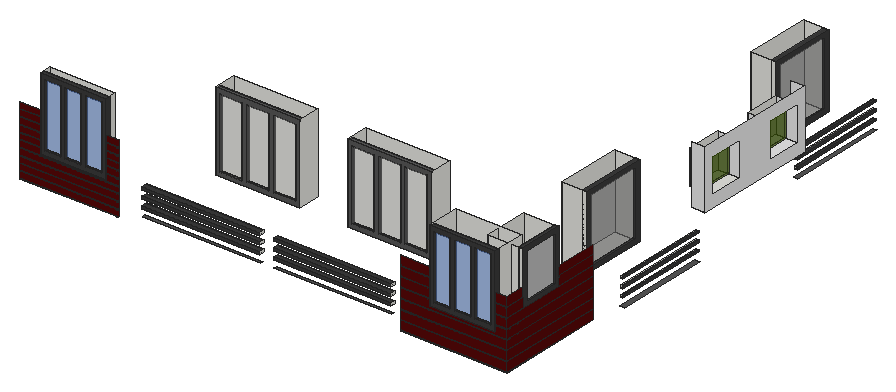
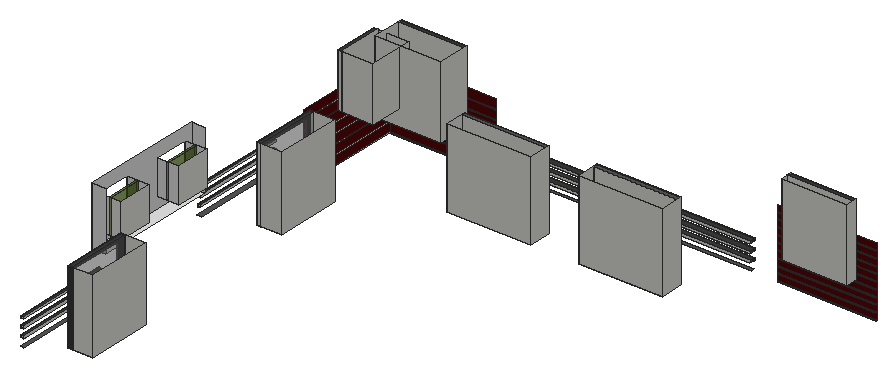
# SketchUp Ruby script. Lengths in inches.
U = 1.inch
M = Sketchup.active_model
def pt(a) = Geom::Point3d.new(a.map { |v| v * U })
def face(e, loops, mat)
  f = e.add_face(loops[0].map { |a| pt(a) })
  loops[1..].each { |l| e.add_face(l.map { |a| pt(a) }).erase! }
  f.material = f.back_material = mat if mat
  f
end
# faces: each face lists its corners as indices into pts; further lists are holes
def faces(e, pts, list, mat = nil) = list.each { |f| face(e, (f[0].is_a?(Array) ? f : [f]).map { |l| l.map { |i| pts[i] } }, mat) }
# xy, xz, yz: faces in a plane at the given z, y or x. An outline is a flat list of corners, or four numbers for a rectangle; further outlines are holes
def ring(l) = l.size == 4 ? [[l[0], l[1]], [l[2], l[1]], [l[2], l[3]], [l[0], l[3]]] : l.each_slice(2).to_a
def flat(e, list, mat, &to3) = list.each { |f| face(e, (f[0].is_a?(Array) ? f : [f]).map { |l| ring(l).map { |u, v| to3.(u, v) } }, mat) }
def xy(e, z, list, mat = nil) = flat(e, list, mat) { |x, y| [x, y, z] }
def xz(e, y, list, mat = nil) = flat(e, list, mat) { |x, z| [x, y, z] }
def yz(e, x, list, mat = nil) = flat(e, list, mat) { |y, z| [x, y, z] }
def lines(e, pts, list) = list.each { |a, b| e.add_line(pt(pts[a]), pt(pts[b])) }
# prism: a flat outline (further loops are holes) pulled along v
def prism(e, loops, v, mat = nil)
  f = face(e, loops, mat); d = Geom::Vector3d.new(v.map { |x| x * U })
  f.pushpull(f.normal.samedirection?(d) ? d.length : -d.length)
end
def box(e, o, s, mat = nil) = prism(e, [[o, [o[0] + s[0], o[1], o[2]], [o[0] + s[0], o[1] + s[1], o[2]], [o[0], o[1] + s[1], o[2]]]], [0, 0, s[2]], mat)
def at(x, y, z, deg = 0) = Geom::Transformation.translation(pt([x, y, z])) * Geom::Transformation.rotation(ORIGIN, Z_AXIS, deg.degrees)
def axes(o, x, y, z) = Geom::Transformation.new([*x, 0, *y, 0, *z, 0, *pt(o).to_a, 1])
def part(name) = M.definitions.add(name)
# library, detail: a bought-in or finely detailed component or shape, given as its bounding box
def library(name, o, s) = part(name).tap { |d| box(d.entities, o, s) }
def detail(e, o, s) = box(e.add_group.entities, o, s)
def put(e, d, t, mat = nil) = e.add_instance(d, t).tap { |i| i.material = mat if mat }
def group(e, t, mat = nil) = e.add_group.tap { |g| g.transformation = t; g.material = mat if mat }.entities
root = M.entities
M.materials.add("Generic").color = [86, 8, 8]
M.materials.add("Generic\#5").color = [230, 230, 230]
M.materials.add("[Color M06]").color = [86, 86, 86]
M.materials.add("[Color M07]").color = [58, 58, 58]
M.materials.add("[Mirror 01]").color = [185, 185, 185]
M.materials.add("[Mirror 02]1").color = [226, 226, 226]
M.materials["[Mirror 02]1"].alpha = 0.26
M.materials.add("[Translucent Glass Blue]").color = [100, 149, 237]
M.materials["[Translucent Glass Blue]"].alpha = 0.5
M.materials.add("[Translucent Glass Dark Green]").color = [62, 91, 5]
M.materials["[Translucent Glass Dark Green]"].alpha = 0.5
M.materials.add("[Translucent Glass Gray]").color = [127, 127, 127]
M.materials["[Translucent Glass Gray]"].alpha = 0.35
c1 = part("Group\#5")
xy(c1.entities,0,[[0,0,6,92.0625]],"[Color M07]")
xy(c1.entities,6.58,[[3,6.58,6,85.48]],"[Color M07]")
xy(c1.entities,96.73,[[3,6.58,6,85.48]],"[Color M07]")
xy(c1.entities,103.3125,[[0,0,6,92.0625]],"[Color M07]")
xz(c1.entities,0,[[0,0,6,103.3125]],"[Color M07]")
xz(c1.entities,6.58,[[3,6.58,6,96.73]],"[Color M07]")
xz(c1.entities,85.48,[[3,6.58,6,96.73]],"[Color M07]")
xz(c1.entities,92.0625,[[0,0,6,103.3125]],"[Color M07]")
yz(c1.entities,0,[[0,0,92.0625,103.3125]],"[Translucent Glass Gray]")
yz(c1.entities,3,[[6.58,6.58,85.48,96.73]],"[Translucent Glass Gray]")
yz(c1.entities,6,[[[0,0,92.0625,103.3125],[6.58,6.58,85.48,96.73]]],"[Color M07]")
c2 = part("Group\#4")
xy(c2.entities,0,[[0,0,117.75,6]],"[Color M06]")
xy(c2.entities,6.37,[[6.37,0,37.125,3],[43.5,0,74.25,3],[80.625,0,111.38,3]],"[Color M06]")
xy(c2.entities,103.75,[[6.37,0,37.125,3],[43.5,0,74.25,3],[80.625,0,111.38,3]],"[Color M06]")
xy(c2.entities,110.125,[[0,0,117.75,6]],"[Color M06]")
xz(c2.entities,0,[[[0,0,117.75,110.125],[6.37,6.37,37.125,103.75],[80.625,6.37,111.38,103.75],[43.5,6.37,74.25,103.75]]],"[Color M06]")
xz(c2.entities,3,[[6.37,6.37,37.125,103.75],[43.5,6.37,74.25,103.75],[80.625,6.37,111.38,103.75]],"[Mirror 02]1")
xz(c2.entities,6,[[0,0,117.75,110.125]])
yz(c2.entities,0,[[0,0,6,110.125]],"[Color M06]")
yz(c2.entities,6.37,[[0,6.37,3,103.75]],"[Color M06]")
yz(c2.entities,37.125,[[0,6.37,3,103.75]],"[Color M06]")
yz(c2.entities,43.5,[[0,6.37,3,103.75]],"[Color M06]")
yz(c2.entities,74.25,[[0,6.37,3,103.75]],"[Color M06]")
yz(c2.entities,80.625,[[0,6.37,3,103.75]],"[Color M06]")
yz(c2.entities,111.38,[[0,6.37,3,103.75]],"[Color M06]")
yz(c2.entities,117.75,[[0,0,6,110.125]],"[Color M06]")
c3 = part("Group\#2")
xy(c3.entities,0,[[0,0,91.6875,6]],"[Color M07]")
xy(c3.entities,6.1,[[6.1,0,28.53,3],[34.63,0,57.06,3],[63.16,0,85.59,3]],"[Color M07]")
xy(c3.entities,95.34,[[6.1,0,28.53,3],[34.63,0,57.06,3],[63.16,0,85.59,3]],"[Color M07]")
xy(c3.entities,101.4375,[[0,0,91.6875,6]],"[Color M07]")
xz(c3.entities,0,[[[0,0,91.6875,101.4375],[34.63,6.1,57.06,95.34],[63.16,6.1,85.59,95.34],[6.1,6.1,28.53,95.34]]],"[Color M07]")
xz(c3.entities,3,[[6.1,6.1,28.53,95.34],[34.63,6.1,57.06,95.34],[63.16,6.1,85.59,95.34]],"[Translucent Glass Blue]")
xz(c3.entities,6,[[0,0,91.6875,101.4375]])
yz(c3.entities,0,[[0,0,6,101.4375]],"[Color M07]")
yz(c3.entities,6.1,[[0,6.1,3,95.34]],"[Color M07]")
yz(c3.entities,28.53,[[0,6.1,3,95.34]],"[Color M07]")
yz(c3.entities,34.63,[[0,6.1,3,95.34]],"[Color M07]")
yz(c3.entities,57.06,[[0,6.1,3,95.34]],"[Color M07]")
yz(c3.entities,63.16,[[0,6.1,3,95.34]],"[Color M07]")
yz(c3.entities,85.59,[[0,6.1,3,95.34]],"[Color M07]")
yz(c3.entities,91.6875,[[0,0,6,101.4375]],"[Color M07]")
c4 = part("Group\#3")
xy(c4.entities,0,[[0,0,6,62.6875]],"[Color M07]")
xy(c4.entities,6.1,[[3,6.1,6,56.59]],"[Color M07]")
xy(c4.entities,69.52,[[3,6.1,6,56.59]],"[Color M07]")
xy(c4.entities,75.625,[[0,0,6,62.6875]],"[Color M07]")
xz(c4.entities,0,[[0,0,6,75.625]],"[Color M07]")
xz(c4.entities,6.1,[[3,6.1,6,69.52]],"[Color M07]")
xz(c4.entities,56.59,[[3,6.1,6,69.52]],"[Color M07]")
xz(c4.entities,62.6875,[[0,0,6,75.625]],"[Color M07]")
yz(c4.entities,0,[[0,0,62.6875,75.625]])
yz(c4.entities,3,[[6.1,6.1,56.59,69.52]],"[Mirror 01]")
yz(c4.entities,6,[[[0,0,62.6875,75.625],[6.1,6.1,56.59,69.52]]],"[Color M07]")
c5 = part("Group\#1")
box(c5.entities,[0,0,0],[3,48.3125,48.3125],"[Translucent Glass Dark Green]")
xy(root,213.125,[[549.5625,113.625,698.4375,113.92],[698.14,113.92,698.4375,263.625]])
xy(root,214.125,[[549.5625,113.625,698.4375,113.92],[698.14,113.92,698.4375,263.625]])
xy(root,217,[[16.6875,113.625,154.5,113.92]])
xy(root,218,[[16.6875,113.625,154.5,113.92]])
xy(root,225.3125,[[183.5625,119.625,347.9375,123.625],[367.1875,119.625,531.5625,123.625]],"[Color M06]")
xy(root,226.6875,[[16.6875,113.625,154.5,113.92],[549.5625,113.625,698.4375,113.92],[698.14,113.92,698.4375,263.625]])
xy(root,227.6875,[[16.6875,113.625,154.5,113.92],[549.5625,113.625,698.4375,113.92],[698.14,113.92,698.4375,263.625]])
xy(root,231.3125,[[721.6875,281.625,728.4375,413.625],[691.25,624.8125,695.75,762.8125]],"[Color M06]")
xy(root,235.82,[[183.5625,118.5,347.9375,125.9375],[367.1875,118.5,531.5625,125.9375]],"[Color M07]")
xy(root,236.375,[[16.6875,113.625,154.5,113.92]])
xy(root,237.375,[[16.6875,113.625,154.5,113.92]])
xy(root,237.48,[[621.0625,306.16,656.0625,398.23]])
xy(root,239.63,[[183.5625,118.5,347.9375,125.9375],[367.1875,118.5,531.5625,125.9375]],"[Color M07]")
xy(root,240.25,[[549.5625,113.625,698.4375,113.92],[698.14,113.92,698.4375,263.625]])
xy(root,241.25,[[549.5625,113.625,698.4375,113.92],[698.14,113.92,698.4375,263.625]])
xy(root,241.4,[[205.67,219.4375,323.42,251.5625],[390.3,219.4375,508.05,251.5625]])
xy(root,241.63,[[606.125,655.17,641.125,747.23]])
xy(root,242.42,[[691.43,624.8125,695.61,762.8125]],"[Color M07]")
xy(root,242.55,[[722.9,281.625,726.28,413.625]],"[Color M07]")
xy(root,245.67,[[722.9,281.625,726.28,413.625]],"[Color M07]")
xy(root,245.74,[[691.43,624.8125,695.61,762.8125]],"[Color M07]")
xy(root,246.0625,[[16.6875,113.625,154.5,113.92]])
xy(root,247.0625,[[16.6875,113.625,154.5,113.92]])
xy(root,247.82,[[183.5625,118.5,347.9375,125.9375],[367.1875,118.5,531.5625,125.9375]],"[Color M07]")
xy(root,251.63,[[183.5625,118.5,347.9375,125.9375],[367.1875,118.5,531.5625,125.9375]],"[Color M07]")
xy(root,253.8125,[[549.5625,113.625,698.4375,113.92],[698.14,113.92,698.4375,263.625]])
xy(root,254.42,[[691.43,624.8125,695.61,762.8125]],"[Color M07]")
xy(root,254.55,[[722.9,281.625,726.28,413.625]],"[Color M07]")
xy(root,254.8125,[[549.5625,113.625,698.4375,113.92],[698.14,113.92,698.4375,263.625]])
xy(root,255.75,[[16.6875,113.625,154.5,113.92]])
xy(root,256.75,[[16.6875,113.625,154.5,113.92]])
xy(root,257.67,[[722.9,281.625,726.28,413.625]],"[Color M07]")
xy(root,257.74,[[691.43,624.8125,695.61,762.8125]],"[Color M07]")
xy(root,258.24,[[44.83,113.625,136.51,130.0625]])
xy(root,258.68,[[589.83,113.625,681.51,159.375]])
xy(root,259.82,[[183.5625,118.5,347.9375,125.9375],[367.1875,118.5,531.5625,125.9375]],"[Color M07]")
xy(root,263.63,[[183.5625,118.5,347.9375,125.9375],[367.1875,118.5,531.5625,125.9375]],"[Color M07]")
xy(root,265.4375,[[16.6875,113.625,44.83,113.625,44.83,113.93,16.6875,113.92],[136.51,113.625,154.5,113.625,154.5,113.92,136.51,113.93]])
xy(root,266.36,[[722.9,281.625,726.28,413.625]],"[Color M07]")
xy(root,266.42,[[691.43,624.8125,695.61,762.8125]],"[Color M07]")
xy(root,266.4375,[[16.6875,113.625,16.6875,113.92,44.83,113.93,44.83,113.625],[136.51,113.625,136.51,113.93,154.5,113.92,154.5,113.625]])
xy(root,267.375,[[549.5625,113.625,589.83,113.625,589.83,113.93,549.5625,113.92],[681.51,113.625,698.4375,113.625,698.4375,113.92,698.14,113.92,681.51,113.93],[698.14,113.92,698.4375,263.625]])
xy(root,268.375,[[549.5625,113.625,549.5625,113.92,589.83,113.93,589.83,113.625],[681.51,113.625,681.51,113.93,698.14,113.92,698.4375,113.92,698.4375,113.625],[698.14,113.92,698.4375,263.625]])
xy(root,269.49,[[722.9,281.625,726.28,413.625]],"[Color M07]")
xy(root,269.74,[[691.43,624.8125,695.61,762.8125]],"[Color M07]")
xy(root,275.125,[[16.6875,113.625,44.83,113.92],[136.51,113.625,154.5,113.92]])
xy(root,276.125,[[16.6875,113.625,44.83,113.92],[136.51,113.625,154.5,113.92]])
xy(root,279.02,[[698.4375,436.65,717.1875,610.59]],"Generic\#5")
xy(root,280.9375,[[549.5625,113.625,589.83,113.625,589.83,113.93,549.5625,113.92],[681.51,113.625,698.4375,113.625,698.4375,113.92,697.84,113.92,681.51,113.93],[697.84,113.92,698.4375,263.625]])
xy(root,281.61,[[697.84,141.33,698.14,204.02]])
xy(root,281.9375,[[549.5625,113.625,549.5625,113.92,589.83,113.93,589.83,113.625],[681.51,113.625,681.51,113.93,697.84,113.92,698.4375,113.92,698.4375,113.625],[697.84,113.92,698.4375,141.33],[697.84,204.02,698.4375,263.625]])
xy(root,284.8125,[[16.6875,113.625,44.83,113.92],[136.51,113.625,154.5,113.92]])
xy(root,285.8125,[[16.6875,113.625,44.83,113.92],[136.51,113.625,154.5,113.92]])
xy(root,294.5,[[16.6875,113.625,44.83,113.92],[136.51,113.625,154.5,113.92],[549.5625,113.625,589.83,113.625,589.83,113.93,549.5625,113.92],[681.51,113.625,698.4375,113.625,698.4375,113.92,698.14,113.92,681.51,113.93],[698.14,113.92,698.4375,141.33],
  [698.14,204.02,698.4375,263.625]])
xy(root,295.43,[[686.125,448.93,717.1875,497.24]])
xy(root,295.43,[[686.125,549.8,717.1875,598.12]],"Generic\#5")
xy(root,295.5,[[16.6875,113.625,44.83,113.92],[136.51,113.625,154.5,113.92],[549.5625,113.625,549.5625,113.92,589.83,113.93,589.83,113.625],[681.51,113.625,681.51,113.93,698.14,113.92,698.4375,113.92,698.4375,113.625],[698.14,113.92,698.4375,141.33],
  [698.14,204.02,698.4375,263.625]])
xy(root,304.1875,[[16.6875,113.625,44.83,113.92],[136.51,113.625,154.5,113.92]])
xy(root,305.1875,[[16.6875,113.625,44.83,113.92],[136.51,113.625,154.5,113.92]])
xz(root,113.625,[[549.5625,214.125,698.4375,226.6875],[16.6875,218,154.5,226.6875],[16.6875,227.6875,154.5,236.375],[549.5625,227.6875,698.4375,240.25],[16.6875,237.375,154.5,246.0625],
  [549.5625,241.25,698.4375,253.8125],[16.6875,247.0625,154.5,255.75],[549.5625,254.8125,698.4375,254.8125,698.4375,267.375,681.51,267.375,681.51,258.68,589.83,258.68,589.83,267.375,549.5625,267.375],[16.6875,256.75,154.5,256.75,154.5,265.4375,136.51,265.4375,136.51,258.24,44.83,258.24,44.83,265.4375,16.6875,265.4375],[16.6875,266.4375,44.83,275.125],
  [136.51,266.4375,154.5,275.125],[549.5625,268.375,589.83,280.9375],[681.51,268.375,698.4375,280.9375],[16.6875,276.125,44.83,284.8125],[136.51,276.125,154.5,284.8125],
  [549.5625,281.9375,589.83,294.5],[681.51,281.9375,698.4375,294.5],[16.6875,285.8125,44.83,294.5],[136.51,285.8125,154.5,294.5],[16.6875,295.5,44.83,304.1875],
  [136.51,295.5,154.5,304.1875],[549.5625,295.5,589.83,308.0625],[681.51,295.5,698.4375,308.0625],[16.6875,305.1875,44.83,313.875],[136.51,305.1875,154.5,313.875]],"Generic")
xz(root,113.92,[[549.5625,213.125,698.14,214.125],[16.6875,217,154.5,218],[16.6875,226.6875,154.5,227.6875],[549.5625,226.6875,698.14,227.6875],[16.6875,236.375,154.5,237.375],
  [549.5625,240.25,698.14,241.25],[16.6875,246.0625,154.5,247.0625],[549.5625,253.8125,698.14,254.8125],[16.6875,255.75,154.5,256.75],[16.6875,275.125,44.83,276.125],
  [136.51,275.125,154.5,276.125],[16.6875,284.8125,44.83,285.8125],[136.51,284.8125,154.5,285.8125],[16.6875,294.5,44.83,295.5],[136.51,294.5,154.5,295.5],
  [16.6875,304.1875,44.83,305.1875],[136.51,304.1875,154.5,305.1875]])
xz(root,118.5,[[183.5625,235.82,347.9375,239.63],[367.1875,235.82,531.5625,239.63],[183.5625,247.82,347.9375,251.63],[367.1875,247.82,531.5625,251.63],[183.5625,259.82,347.9375,263.63],
  [367.1875,259.82,531.5625,263.63]],"[Color M07]")
xz(root,125.9375,[[183.5625,235.82,347.9375,239.63],[367.1875,235.82,531.5625,239.63],[183.5625,247.82,347.9375,251.63],[367.1875,247.82,531.5625,251.63],[183.5625,259.82,347.9375,263.63],
  [367.1875,259.82,531.5625,263.63]])
xz(root,130.0625,[[44.83,258.24,136.51,359.68]])
xz(root,141.33,[[648.625,280.49,698.4375,281.61,697.84,281.61,697.84,281.9375,698.4375,281.9375,698.4375,294.5,698.14,294.5,698.14,295.5,698.4375,295.5,698.4375,308.0625,698.14,308.0625,698.14,309.0625,698.4375,309.0625,698.4375,321.625,698.14,321.625,698.14,322.625,698.4375,322.625,698.4375,335.1875,698.14,335.1875,698.14,336.1875,698.4375,336.1875,698.4375,348.75,698.14,348.75,698.14,349.75,698.4375,349.75,698.4375,356.11,648.625,356.11],[697.84,281.61,698.4375,281.9375],[698.14,294.5,698.4375,295.5]])
xz(root,159.375,[[589.83,258.68,681.51,360.11]])
xz(root,204.02,[[648.625,280.49,648.625,356.11,698.4375,356.11,698.4375,349.75,698.14,349.75,698.14,348.75,698.4375,348.75,698.4375,336.1875,698.14,336.1875,698.14,335.1875,698.4375,335.1875,698.4375,322.625,698.14,322.625,698.14,321.625,698.4375,321.625,698.4375,309.0625,698.14,309.0625,698.14,308.0625,698.4375,308.0625,698.4375,295.5,698.14,295.5,698.14,294.5,698.4375,294.5,698.4375,281.9375,697.84,281.9375,697.84,281.61,698.4375,281.61],[697.84,281.61,698.4375,281.9375],[698.14,294.5,698.4375,295.5]])
xz(root,251.5625,[[205.67,241.4,323.42,351.52],[390.3,241.4,508.05,351.52]])
xz(root,263.625,[[698.14,213.125,698.4375,214.125],[698.14,226.6875,698.4375,227.6875],[698.14,240.25,698.4375,241.25],[698.14,253.8125,698.4375,254.8125],[698.14,267.375,698.4375,268.375],
  [697.84,280.9375,698.4375,281.9375],[698.14,294.5,698.4375,295.5]])
xz(root,306.16,[[621.0625,237.48,656.0625,340.79]])
xz(root,398.23,[[621.0625,237.48,656.0625,340.79]])
xz(root,413.625,[[722.9,242.55,726.28,245.67],[722.9,254.55,726.28,257.67],[722.9,266.36,726.28,269.49]])
xz(root,436.65,[[698.4375,279.02,717.1875,361.33]],"Generic\#5")
xz(root,448.93,[[686.125,295.43,717.1875,343.74]],"Generic\#5")
xz(root,497.24,[[686.125,295.43,717.1875,343.74]],"Generic\#5")
xz(root,549.8,[[686.125,295.43,717.1875,343.74]],"Generic\#5")
xz(root,598.12,[[686.125,295.43,717.1875,343.74]],"Generic\#5")
xz(root,610.59,[[698.4375,279.02,717.1875,361.33]],"Generic\#5")
xz(root,655.17,[[606.125,241.63,641.125,344.94]])
xz(root,747.23,[[606.125,241.63,641.125,344.94]])
xz(root,762.8125,[[691.43,242.42,695.61,245.74],[691.43,254.42,695.61,257.74],[691.43,266.42,695.61,269.74]])
yz(root,44.83,[[113.625,258.24,130.0625,258.24,130.0625,359.68,113.625,359.68,113.625,353.625,113.93,353.625,113.93,352.625,113.625,352.625,113.625,343.9375,113.93,343.9375,113.93,342.9375,113.625,342.9375,113.625,334.25,113.92,334.25,113.92,333.25,113.625,333.25,113.625,324.5625,113.92,324.5625,113.92,323.5625,113.625,323.5625,113.625,314.875,113.92,314.875,113.92,313.875,113.625,313.875,113.625,305.1875,113.92,305.1875,113.92,304.1875,113.625,304.1875,113.625,295.5,113.92,295.5,113.92,294.5,113.625,294.5,113.625,285.8125,113.92,285.8125,113.92,284.8125,113.625,284.8125,113.625,276.125,113.92,276.125,113.92,275.125,113.625,275.125,113.625,266.4375,113.93,266.4375,113.93,265.4375,113.625,265.4375]])
yz(root,136.51,[[113.625,258.24,113.625,265.4375,113.93,265.4375,113.93,266.4375,113.625,266.4375,113.625,275.125,113.92,275.125,113.92,276.125,113.625,276.125,113.625,284.8125,113.92,284.8125,113.92,285.8125,113.625,285.8125,113.625,294.5,113.92,294.5,113.92,295.5,113.625,295.5,113.625,304.1875,113.92,304.1875,113.92,305.1875,113.625,305.1875,113.625,313.875,113.92,313.875,113.92,314.875,113.625,314.875,113.625,323.5625,113.92,323.5625,113.92,324.5625,113.625,324.5625,113.625,333.25,113.92,333.25,113.92,334.25,113.625,334.25,113.625,342.9375,113.93,342.9375,113.93,343.9375,113.625,343.9375,113.625,352.625,113.93,352.625,113.93,353.625,113.625,353.625,113.625,359.68,130.0625,359.68,130.0625,258.24]])
yz(root,154.5,[[113.625,217,113.92,218],[113.625,226.6875,113.92,227.6875],[113.625,236.375,113.92,237.375],[113.625,246.0625,113.92,247.0625],[113.625,255.75,113.92,256.75],
  [113.625,265.4375,113.92,266.4375],[113.625,275.125,113.92,276.125],[113.625,284.8125,113.92,285.8125],[113.625,294.5,113.92,295.5],[113.625,304.1875,113.92,305.1875]])
yz(root,205.67,[[219.4375,241.4,251.5625,351.52]])
yz(root,323.42,[[219.4375,241.4,251.5625,351.52]])
yz(root,347.9375,[[118.5,235.82,125.9375,239.63],[118.5,247.82,125.9375,251.63],[118.5,259.82,125.9375,263.63]])
yz(root,390.3,[[219.4375,241.4,251.5625,351.52]])
yz(root,508.05,[[219.4375,241.4,251.5625,351.52]])
yz(root,531.5625,[[118.5,235.82,125.9375,239.63],[118.5,247.82,125.9375,251.63],[118.5,259.82,125.9375,263.63]])
yz(root,549.5625,[[113.625,213.125,113.92,214.125],[113.625,226.6875,113.92,227.6875],[113.625,240.25,113.92,241.25],[113.625,253.8125,113.92,254.8125],[113.625,267.375,113.92,268.375],
  [113.625,280.9375,113.92,281.9375],[113.625,294.5,113.92,295.5]])
yz(root,589.83,[[113.625,258.68,159.375,258.68,159.375,360.11,113.625,360.11,113.625,349.75,113.93,349.75,113.93,348.75,113.625,348.75,113.625,336.1875,113.93,336.1875,113.93,335.1875,113.625,335.1875,113.625,322.625,113.92,322.625,113.93,321.625,113.625,321.625,113.625,309.0625,113.93,309.0625,113.93,308.0625,113.625,308.0625,113.625,295.5,113.93,295.5,113.93,294.5,113.625,294.5,113.625,281.9375,113.93,281.9375,113.93,280.9375,113.625,280.9375,113.625,268.375,113.93,268.375,113.93,267.375,113.625,267.375]])
yz(root,606.125,[[655.17,241.63,747.23,344.94]])
yz(root,621.0625,[[306.16,237.48,398.23,340.79]])
yz(root,648.625,[[141.33,280.49,204.02,356.11]])
yz(root,681.51,[[113.625,258.68,113.625,267.375,113.93,267.375,113.93,268.375,113.625,268.375,113.625,280.9375,113.93,280.9375,113.93,281.9375,113.625,281.9375,113.625,294.5,113.93,294.5,113.93,295.5,113.625,295.5,113.625,308.0625,113.93,308.0625,113.93,309.0625,113.625,309.0625,113.625,321.625,113.93,321.625,113.92,322.625,113.625,322.625,113.625,335.1875,113.93,335.1875,113.93,336.1875,113.625,336.1875,113.625,348.75,113.93,348.75,113.93,349.75,113.625,349.75,113.625,360.11,159.375,360.11,159.375,258.68]])
yz(root,686.125,[[448.93,295.43,497.24,343.74],[549.8,295.43,598.12,343.74]])
yz(root,691.43,[[624.8125,242.42,762.8125,245.74],[624.8125,254.42,762.8125,257.74],[624.8125,266.42,762.8125,269.74]])
yz(root,695.61,[[624.8125,242.42,762.8125,245.74],[624.8125,254.42,762.8125,257.74],[624.8125,266.42,762.8125,269.74]],"[Color M07]")
yz(root,697.84,[[113.92,280.9375,113.92,281.9375,141.33,281.9375,141.33,281.61,204.02,281.61,204.02,281.9375,263.625,281.9375,263.625,280.9375]])
yz(root,698.14,[[113.92,213.125,263.625,214.125],[113.92,226.6875,263.625,227.6875],[113.92,240.25,263.625,241.25],[113.92,253.8125,263.625,254.8125],[113.92,267.375,263.625,268.375],
  [113.92,280.9375,263.625,280.9375,263.625,281.9375,204.02,281.9375,204.02,281.61,141.33,281.61,141.33,281.9375,113.92,281.9375],[113.92,294.5,141.33,295.5],[204.02,294.5,263.625,295.5]])
yz(root,698.4375,[[113.625,214.125,263.625,226.6875],[113.625,227.6875,263.625,240.25],[113.625,241.25,263.625,253.8125],[113.625,254.8125,263.625,267.375],[113.625,268.375,263.625,280.9375],
  [113.625,281.9375,141.33,294.5],[204.02,281.9375,263.625,294.5],[113.625,295.5,141.33,308.0625],[204.02,295.5,263.625,308.0625]],"Generic")
yz(root,717.1875,[[[436.65,279.02,610.59,361.33],[448.93,295.43,497.24,343.74],[549.8,295.43,598.12,343.74]]],"Generic\#5")
yz(root,722.9,[[281.625,242.55,413.625,245.67],[281.625,254.55,413.625,257.67],[281.625,266.36,413.625,269.49]])
yz(root,726.28,[[281.625,242.55,413.625,245.67],[281.625,254.55,413.625,257.67],[281.625,266.36,413.625,269.49]],"[Color M07]")
p = [[16.6875,113.92,265.4375],[44.83,113.93,265.4375],[44.83,113.93,266.4375],[16.6875,113.92,266.4375],[154.5,113.92,265.4375],[154.5,113.92,266.4375],
  [136.51,113.93,266.4375],[136.51,113.93,265.4375],[549.5625,113.92,267.375],[589.83,113.93,267.375],[589.83,113.93,268.375],[549.5625,113.92,268.375],
  [681.51,113.93,267.375],[698.14,113.92,267.375],[698.14,113.92,268.375],[681.51,113.93,268.375],[549.5625,113.92,280.9375],[589.83,113.93,280.9375],
  [589.83,113.93,281.9375],[549.5625,113.92,281.9375],[697.84,113.92,280.9375],[681.51,113.93,280.9375],[681.51,113.93,281.9375],[697.84,113.92,281.9375],
  [549.5625,113.92,294.5],[589.83,113.93,294.5],[589.83,113.93,295.5],[549.5625,113.92,295.5],[681.51,113.93,294.5],[698.14,113.92,294.5],
  [698.14,113.92,295.5],[681.51,113.93,295.5],[531.5625,121.625,237.3125],[367.1875,121.625,237.3125],[531.5625,121.625,249.3125],[367.1875,121.625,249.3125],
  [531.5625,121.625,261.3125],[367.1875,121.625,261.3125],[347.9375,121.625,237.3125],[183.5625,121.625,237.3125],[347.9375,121.625,249.3125],[183.5625,121.625,249.3125],
  [347.9375,121.625,261.3125],[183.5625,121.625,261.3125],[693.5,762.8125,243.3125],[693.5,624.8125,243.3125],[693.5,762.8125,255.3125],[693.5,624.8125,255.3125],
  [693.5,762.8125,267.3125],[693.5,624.8125,267.3125],[725.0625,413.625,243.3125],[725.0625,281.625,243.3125],[725.0625,413.625,255.3125],[725.0625,281.625,255.3125],
  [725.0625,413.625,267.3125],[725.0625,281.625,267.3125]]
faces(root,p,[[0,1,2,3],[4,5,6,7],[8,9,10,11],[12,13,14,15],[16,17,18,19],[20,21,22,23],[24,25,26,27],[28,29,30,31]])
lines(root,p,[[32,33],[34,35],[36,37],[38,39],[40,41],[42,43],[44,45],[46,47],[48,49],[50,51],[52,53],[54,55]])
put(root,c1,at(650.0625,306.16,237.48))
put(root,c2,at(205.67,219.4375,241.4))
put(root,c2,at(390.3,219.4375,241.4))
put(root,c1,at(635.125,655.17,241.63))
put(root,c3,at(44.83,113.625,258.24))
put(root,c3,at(589.83,113.625,258.68))
put(root,c4,at(692.4375,141.33,281.61))
put(root,c5,at(699.6875,448.93,295.43))
put(root,c5,at(699.6875,549.8,295.43))
